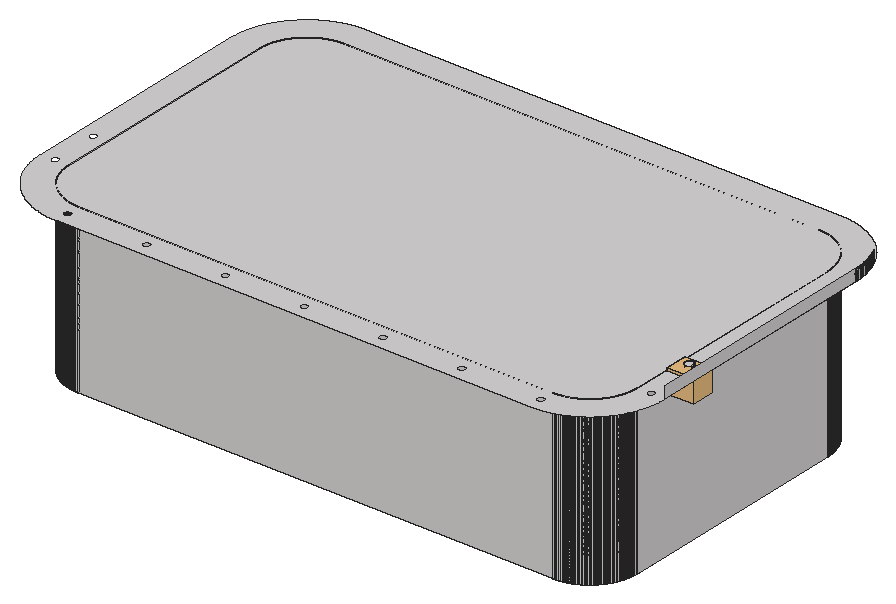
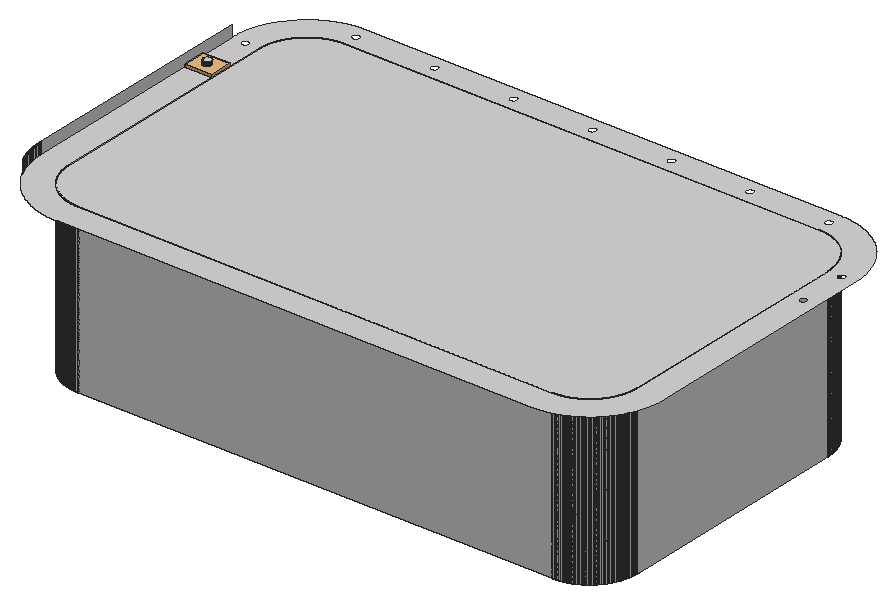
# SketchUp Ruby script. Lengths in inches.
U = 1.inch
M = Sketchup.active_model
def pt(a) = Geom::Point3d.new(a.map { |v| v * U })
def face(e, loops, mat)
  f = e.add_face(loops[0].map { |a| pt(a) })
  loops[1..].each { |l| e.add_face(l.map { |a| pt(a) }).erase! }
  f.material = f.back_material = mat if mat
  f
end
# faces: each face lists its corners as indices into pts; further lists are holes
def faces(e, pts, list, mat = nil) = list.each { |f| face(e, (f[0].is_a?(Array) ? f : [f]).map { |l| l.map { |i| pts[i] } }, mat) }
# xy, xz, yz: faces in a plane at the given z, y or x. An outline is a flat list of corners, or four numbers for a rectangle; further outlines are holes
def ring(l) = l.size == 4 ? [[l[0], l[1]], [l[2], l[1]], [l[2], l[3]], [l[0], l[3]]] : l.each_slice(2).to_a
def flat(e, list, mat, &to3) = list.each { |f| face(e, (f[0].is_a?(Array) ? f : [f]).map { |l| ring(l).map { |u, v| to3.(u, v) } }, mat) }
def xy(e, z, list, mat = nil) = flat(e, list, mat) { |x, y| [x, y, z] }
def xz(e, y, list, mat = nil) = flat(e, list, mat) { |x, z| [x, y, z] }
def yz(e, x, list, mat = nil) = flat(e, list, mat) { |y, z| [x, y, z] }
def lines(e, pts, list) = list.each { |a, b| e.add_line(pt(pts[a]), pt(pts[b])) }
# prism: a flat outline (further loops are holes) pulled along v
def prism(e, loops, v, mat = nil)
  f = face(e, loops, mat); d = Geom::Vector3d.new(v.map { |x| x * U })
  f.pushpull(f.normal.samedirection?(d) ? d.length : -d.length)
end
def box(e, o, s, mat = nil) = prism(e, [[o, [o[0] + s[0], o[1], o[2]], [o[0] + s[0], o[1] + s[1], o[2]], [o[0], o[1] + s[1], o[2]]]], [0, 0, s[2]], mat)
def at(x, y, z, deg = 0) = Geom::Transformation.translation(pt([x, y, z])) * Geom::Transformation.rotation(ORIGIN, Z_AXIS, deg.degrees)
def axes(o, x, y, z) = Geom::Transformation.new([*x, 0, *y, 0, *z, 0, *pt(o).to_a, 1])
def part(name) = M.definitions.add(name)
# library, detail: a bought-in or finely detailed component or shape, given as its bounding box
def library(name, o, s) = part(name).tap { |d| box(d.entities, o, s) }
def detail(e, o, s) = box(e.add_group.entities, o, s)
def put(e, d, t, mat = nil) = e.add_instance(d, t).tap { |i| i.material = mat if mat }
def group(e, t, mat = nil) = e.add_group.tap { |g| g.transformation = t; g.material = mat if mat }.entities
root = M.entities
M.materials.add("[Quartz Light Brown]").color = [215, 212, 212]
c1 = library("3",[-5.26,-4.28,-11.86],[13.52,11.56,11.86])
xy(root,480,[[[224.5,282.7,224.01,282.71,223.01,282.75,222.51,282.78,222.02,282.82,221.52,282.86,221.03,282.91,220.53,282.96,220.04,283.03,219.55,283.09,219.06,283.17,218.56,283.25,218.08,283.34,217.59,283.43,217.1,283.53,216.61,283.64,216.13,283.75,215.65,283.87,215.16,284,214.69,284.13,213.73,284.41,213.26,284.5625,212.79,284.72,212.32,284.88,211.38,285.22,210.92,285.41,210.46,285.59,209.54,285.99,209.09,286.19,208.64,286.4,208.19,286.62,207.75,286.84,207.31,287.07,206.43,287.55,206,287.79,205.57,288.04,205.15,288.3,204.72,288.5625,204.3,288.83,203.89,289.11,203.48,289.38,202.66,289.96,202.26,290.25,201.87,290.55,201.47,290.86,201.09,291.17,200.7,291.49,199.94,292.13,199.57,292.46,199.21,292.8,198.84,293.14,198.48,293.48,197.78,294.18,197.4375,294.54,197.1,294.91,196.76,295.27,196.43,295.65,196.1,296.02,195.78,296.4,194.85,297.57,194.55,297.96,194.26,298.37,193.97,298.77,193.68,299.18,193.4,299.59,193.13,300,192.86,300.42,192.6,300.85,192.34,301.27,192.09,301.7,191.85,302.13,191.6,302.57,191.14,303.45,190.92,303.89,190.7,304.34,190.49,304.79,190.29,305.25,190.09,305.7,189.89,306.16,189.71,306.62,189.52,307.08,189.18,308.02,188.86,308.96,188.71,309.43,188.56,309.91,188.43,310.39,188.29,310.87,188.05,311.83,187.9375,312.31,187.83,312.8,187.73,313.29,187.55,314.27,187.39,315.25,187.33,315.74,187.26,316.23,187.21,316.73,187.16,317.22,187.08,318.22,187.05,318.71,187.01,319.71,187,320.2,187,441.2,187.01,441.7,187.03,442.19,187.05,442.69,187.08,443.1875,187.12,443.68,187.16,444.18,187.21,444.67,187.26,445.17,187.33,445.66,187.39,446.15,187.47,446.65,187.55,447.14,187.73,448.11,187.83,448.6,187.9375,449.09,188.05,449.57,188.17,450.05,188.29,450.54,188.43,451.02,188.56,451.49,188.71,451.97,188.86,452.44,189.02,452.92,189.18,453.39,189.35,453.85,189.52,454.32,189.71,454.78,189.89,455.24,190.29,456.16,190.49,456.61,190.7,457.06,190.92,457.51,191.14,457.95,191.6,458.83,191.85,459.27,192.09,459.7,192.34,460.13,192.6,460.56,192.86,460.98,193.13,461.4,193.4,461.8125,193.68,462.22,194.26,463.04,194.55,463.4375,194.85,463.83,195.16,464.23,195.47,464.62,195.78,465,196.1,465.38,196.43,465.76,196.76,466.13,197.1,466.5,197.4375,466.86,197.78,467.22,198.48,467.92,198.84,468.27,199.21,468.61,199.57,468.94,199.94,469.27,200.32,469.6,200.7,469.92,201.09,470.23,201.47,470.54,201.87,470.85,202.26,471.15,202.66,471.44,203.48,472.02,203.89,472.3,204.3,472.57,204.72,472.84,205.15,473.1,205.57,473.36,206.43,473.86,206.87,474.1,207.75,474.56,208.19,474.78,208.64,475,209.54,475.42,210,475.62,210.92,476,211.38,476.18,212.32,476.52,213.26,476.84,213.73,476.99,214.21,477.14,214.69,477.27,215.16,477.41,215.65,477.53,216.13,477.65,216.61,477.76,217.1,477.87,217.59,477.97,218.08,478.06,218.56,478.15,219.06,478.23,219.55,478.31,220.04,478.375,220.53,478.4375,221.03,478.49,221.52,478.54,222.02,478.58,222.51,478.62,223.01,478.65,223.51,478.67,224.01,478.6875,224.5,478.7,464.5,478.7,464.99,478.6875,465.49,478.67,465.99,478.65,466.49,478.62,466.98,478.58,467.48,478.54,467.97,478.49,468.47,478.4375,468.96,478.375,469.45,478.31,469.94,478.23,470.44,478.15,470.92,478.06,471.41,477.97,471.9,477.87,472.39,477.76,472.87,477.65,473.35,477.53,473.84,477.41,474.31,477.27,474.79,477.14,475.27,476.99,475.74,476.84,476.68,476.52,477.62,476.18,478.08,476,479,475.62,479.46,475.42,480.36,475,480.81,474.78,481.25,474.56,482.13,474.1,482.57,473.86,483.43,473.36,483.85,473.1,484.28,472.84,484.7,472.57,485.11,472.3,485.52,472.02,486.34,471.44,486.74,471.15,487.13,470.85,487.53,470.54,487.91,470.23,488.3,469.92,488.68,469.6,489.06,469.27,489.43,468.94,489.79,468.61,490.16,468.27,490.52,467.92,491.22,467.22,491.5625,466.86,491.9,466.5,492.24,466.13,492.57,465.76,492.9,465.38,493.22,465,493.53,464.62,493.84,464.23,494.15,463.83,494.45,463.4375,494.74,463.04,495.32,462.22,495.6,461.8125,495.87,461.4,496.14,460.98,496.4,460.56,496.66,460.13,496.91,459.7,497.15,459.27,497.4,458.83,497.86,457.95,498.08,457.51,498.3,457.06,498.51,456.61,498.71,456.16,499.11,455.24,499.29,454.78,499.48,454.32,499.65,453.85,499.82,453.39,499.98,452.92,500.14,452.44,500.29,451.97,500.44,451.49,500.57,451.02,500.71,450.54,500.83,450.05,500.95,449.57,501.0625,449.09,501.17,448.6,501.27,448.11,501.45,447.14,501.53,446.65,501.61,446.15,501.67,445.66,501.74,445.17,501.79,444.67,501.84,444.18,501.88,443.68,501.92,443.1875,501.95,442.69,501.97,442.19,501.99,441.7,502,441.2,502,320.2,501.99,319.71,501.95,318.71,501.92,318.22,501.84,317.22,501.79,316.73,501.74,316.23,501.67,315.74,501.61,315.25,501.45,314.27,501.27,313.29,501.17,312.8,501.0625,312.31,500.95,311.83,500.71,310.87,500.57,310.39,500.44,309.91,500.29,309.43,500.14,308.96,499.82,308.02,499.48,307.08,499.29,306.62,499.11,306.16,498.91,305.7,498.71,305.25,498.51,304.79,498.3,304.34,498.08,303.89,497.86,303.45,497.4,302.57,497.15,302.13,496.91,301.7,496.66,301.27,496.4,300.85,496.14,300.42,495.87,300,495.6,299.59,495.32,299.18,495.03,298.77,494.74,298.37,494.45,297.96,494.15,297.57,493.22,296.4,492.9,296.02,492.57,295.65,492.24,295.27,491.9,294.91,491.5625,294.54,491.22,294.18,490.52,293.48,490.16,293.14,489.79,292.8,489.43,292.46,489.06,292.13,488.3,291.49,487.91,291.17,487.53,290.86,487.13,290.55,486.74,290.25,486.34,289.96,485.52,289.38,485.11,289.11,484.7,288.83,484.28,288.5625,483.85,288.3,483.43,288.04,483,287.79,482.57,287.55,481.69,287.07,481.25,286.84,480.81,286.62,480.36,286.4,479.91,286.19,479.46,285.99,478.54,285.59,478.08,285.41,477.62,285.22,476.68,284.88,476.21,284.72,475.74,284.5625,475.27,284.41,474.31,284.13,473.84,284,473.35,283.87,472.87,283.75,472.39,283.64,471.9,283.53,471.41,283.43,470.92,283.34,470.44,283.25,469.94,283.17,469.45,283.09,468.96,283.03,468.47,282.96,467.97,282.91,467.48,282.86,466.98,282.82,466.49,282.78,465.99,282.75,464.99,282.71,464.5,282.7],[494.91,342.7,495.0625,342.7,495.22,342.71,495.53,342.77,495.68,342.82,495.82,342.88,495.96,342.95,496.1,343.03,496.23,343.12,496.35,343.22,496.46,343.33,496.56,343.45,496.74,343.71,496.81,343.85,496.87,343.99,496.92,344.14,496.96,344.29,497,344.61,497,344.76,496.99,344.92,496.96,345.08,496.93,345.23,496.88,345.38,496.82,345.52,496.75,345.66,496.67,345.8,496.58,345.93,496.48,346.05,496.37,346.16,496.25,346.26,496.125,346.35,495.99,346.4375,495.85,346.51,495.71,346.57,495.56,346.62,495.41,346.66,495.25,346.69,495.09,346.7,494.9375,346.7,494.78,346.6875,494.625,346.67,494.47,346.63,494.32,346.58,494.18,346.52,494.04,346.45,493.9,346.37,493.77,346.28,493.65,346.18,493.54,346.07,493.44,345.95,493.35,345.83,493.26,345.69,493.19,345.55,493.13,345.41,493.08,345.26,493.04,345.11,493.02,344.95,493,344.8,493,344.64,493.01,344.48,493.04,344.33,493.07,344.17,493.12,344.02,493.18,343.88,493.25,343.74,493.33,343.6,493.42,343.48,493.52,343.36,493.63,343.24,493.75,343.14,493.875,343.05,494.01,342.96,494.15,342.89,494.29,342.83,494.44,342.78,494.59,342.74],[494.91,318.7,495.0625,318.7,495.22,318.71,495.53,318.77,495.68,318.82,495.82,318.88,495.96,318.95,496.1,319.03,496.23,319.12,496.35,319.22,496.46,319.33,496.56,319.45,496.74,319.71,496.81,319.85,496.87,319.99,496.92,320.14,496.96,320.29,497,320.61,497,320.76,496.99,320.92,496.96,321.08,496.93,321.23,496.88,321.38,496.82,321.52,496.75,321.66,496.67,321.8,496.58,321.93,496.48,322.05,496.37,322.16,496.25,322.26,496.125,322.35,495.99,322.4375,495.85,322.51,495.71,322.57,495.56,322.62,495.41,322.66,495.25,322.69,495.09,322.7,494.9375,322.7,494.78,322.6875,494.625,322.67,494.47,322.63,494.32,322.58,494.18,322.52,494.04,322.45,493.9,322.37,493.77,322.28,493.65,322.18,493.54,322.07,493.44,321.95,493.35,321.83,493.26,321.69,493.19,321.55,493.13,321.41,493.08,321.26,493.04,321.11,493.02,320.95,493,320.8,493,320.64,493.01,320.48,493.04,320.33,493.07,320.17,493.12,320.02,493.18,319.88,493.25,319.74,493.33,319.6,493.42,319.48,493.52,319.36,493.63,319.24,493.75,319.14,493.875,319.05,494.01,318.96,494.15,318.89,494.29,318.83,494.44,318.78,494.59,318.74],[224.9375,287.7,225.09,287.7,225.41,287.74,225.56,287.78,225.71,287.83,225.85,287.89,225.99,287.96,226.125,288.05,226.25,288.14,226.37,288.24,226.48,288.36,226.58,288.48,226.67,288.6,226.75,288.74,226.82,288.88,226.88,289.02,226.93,289.17,226.96,289.33,226.99,289.48,227,289.64,227,289.8,226.98,289.95,226.96,290.11,226.92,290.26,226.87,290.41,226.81,290.55,226.74,290.69,226.65,290.83,226.56,290.95,226.46,291.07,226.35,291.18,226.23,291.28,226.1,291.37,225.96,291.45,225.82,291.52,225.68,291.58,225.53,291.63,225.375,291.67,225.22,291.6875,225.0625,291.7,224.91,291.7,224.75,291.69,224.59,291.66,224.44,291.62,224.29,291.57,224.15,291.51,224.01,291.4375,223.875,291.35,223.75,291.26,223.63,291.16,223.52,291.05,223.42,290.93,223.33,290.8,223.25,290.66,223.18,290.52,223.12,290.38,223.07,290.23,223.04,290.08,223.01,289.92,223,289.76,223,289.61,223.04,289.29,223.08,289.14,223.13,288.99,223.19,288.85,223.26,288.71,223.44,288.45,223.54,288.33,223.65,288.22,223.77,288.12,223.9,288.03,224.04,287.95,224.18,287.88,224.32,287.82,224.47,287.77,224.78,287.71],[264.77,287.7,264.93,287.7,265.08,287.72,265.24,287.74,265.39,287.78,265.54,287.83,265.69,287.89,265.82,287.96,265.96,288.05,266.08,288.14,266.2,288.24,266.3125,288.36,266.41,288.48,266.51,288.6,266.59,288.74,266.66,288.88,266.72,289.02,266.76,289.17,266.8,289.33,266.82,289.48,266.83,289.64,266.83,289.8,266.82,289.95,266.79,290.11,266.75,290.26,266.7,290.41,266.64,290.55,266.57,290.69,266.49,290.83,266.29,291.07,266.18,291.18,266.06,291.28,265.93,291.37,265.8,291.45,265.66,291.52,265.51,291.58,265.36,291.63,265.21,291.67,265.05,291.6875,264.9,291.7,264.74,291.7,264.58,291.69,264.43,291.66,264.27,291.62,264.125,291.57,263.98,291.51,263.84,291.4375,263.71,291.35,263.58,291.26,263.46,291.16,263.35,291.05,263.25,290.93,263.16,290.8,263.08,290.66,263.01,290.52,262.95,290.38,262.9,290.23,262.87,290.08,262.83,289.76,262.84,289.61,262.85,289.45,262.875,289.29,262.91,289.14,262.96,288.99,263.02,288.85,263.1,288.71,263.18,288.58,263.27,288.45,263.375,288.33,263.49,288.22,263.61,288.12,263.74,288.03,263.87,287.95,264.01,287.88,264.16,287.82,264.31,287.77,264.61,287.71],[304.6,287.7,304.76,287.7,304.92,287.72,305.07,287.74,305.23,287.78,305.375,287.83,305.52,287.89,305.66,287.96,305.92,288.14,306.04,288.24,306.15,288.36,306.25,288.48,306.34,288.6,306.42,288.74,306.49,288.88,306.55,289.02,306.6,289.17,306.63,289.33,306.65,289.48,306.67,289.64,306.66,289.8,306.65,289.95,306.625,290.11,306.59,290.26,306.54,290.41,306.48,290.55,306.32,290.83,306.23,290.95,306.125,291.07,306.01,291.18,305.89,291.28,305.76,291.37,305.63,291.45,305.49,291.52,305.34,291.58,305.19,291.63,305.04,291.67,304.89,291.6875,304.73,291.7,304.57,291.7,304.42,291.69,304.26,291.66,304.11,291.62,303.96,291.57,303.81,291.51,303.68,291.4375,303.54,291.35,303.42,291.26,303.3,291.16,303.1875,291.05,303.09,290.93,302.99,290.8,302.91,290.66,302.84,290.52,302.78,290.38,302.7,290.08,302.68,289.92,302.67,289.76,302.67,289.61,302.68,289.45,302.71,289.29,302.75,289.14,302.8,288.99,302.86,288.85,302.93,288.71,303.01,288.58,303.11,288.45,303.21,288.33,303.32,288.22,303.44,288.12,303.57,288.03,303.7,287.95,303.84,287.88,303.99,287.82,304.14,287.77,304.29,287.74,304.45,287.71],[344.4375,287.7,344.59,287.7,344.91,287.74,345.06,287.78,345.21,287.83,345.35,287.89,345.49,287.96,345.625,288.05,345.75,288.14,345.87,288.24,345.98,288.36,346.08,288.48,346.17,288.6,346.25,288.74,346.32,288.88,346.38,289.02,346.43,289.17,346.46,289.33,346.49,289.48,346.5,289.64,346.5,289.8,346.48,289.95,346.46,290.11,346.42,290.26,346.37,290.41,346.31,290.55,346.24,290.69,346.15,290.83,346.06,290.95,345.96,291.07,345.85,291.18,345.73,291.28,345.6,291.37,345.46,291.45,345.32,291.52,345.18,291.58,345.03,291.63,344.875,291.67,344.72,291.6875,344.5625,291.7,344.41,291.7,344.25,291.69,344.09,291.66,343.94,291.62,343.79,291.57,343.65,291.51,343.51,291.4375,343.375,291.35,343.25,291.26,343.13,291.16,343.02,291.05,342.92,290.93,342.83,290.8,342.75,290.66,342.68,290.52,342.62,290.38,342.57,290.23,342.54,290.08,342.51,289.92,342.5,289.76,342.5,289.61,342.54,289.29,342.58,289.14,342.63,288.99,342.69,288.85,342.76,288.71,342.94,288.45,343.04,288.33,343.15,288.22,343.27,288.12,343.4,288.03,343.54,287.95,343.68,287.88,343.82,287.82,343.97,287.77,344.28,287.71],[384.27,287.7,384.43,287.7,384.58,287.72,384.74,287.74,384.89,287.78,385.04,287.83,385.19,287.89,385.32,287.96,385.46,288.05,385.58,288.14,385.7,288.24,385.8125,288.36,385.91,288.48,386.01,288.6,386.09,288.74,386.16,288.88,386.22,289.02,386.26,289.17,386.3,289.33,386.32,289.48,386.33,289.64,386.33,289.8,386.32,289.95,386.29,290.11,386.25,290.26,386.2,290.41,386.14,290.55,386.07,290.69,385.99,290.83,385.79,291.07,385.68,291.18,385.56,291.28,385.43,291.37,385.3,291.45,385.16,291.52,385.01,291.58,384.86,291.63,384.71,291.67,384.55,291.6875,384.4,291.7,384.24,291.7,384.08,291.69,383.93,291.66,383.77,291.62,383.625,291.57,383.48,291.51,383.34,291.4375,383.21,291.35,383.08,291.26,382.96,291.16,382.85,291.05,382.75,290.93,382.66,290.8,382.58,290.66,382.51,290.52,382.45,290.38,382.4,290.23,382.37,290.08,382.33,289.76,382.34,289.61,382.35,289.45,382.375,289.29,382.41,289.14,382.46,288.99,382.52,288.85,382.6,288.71,382.68,288.58,382.77,288.45,382.875,288.33,382.99,288.22,383.11,288.12,383.24,288.03,383.37,287.95,383.51,287.88,383.66,287.82,383.81,287.77,384.11,287.71],[424.1,287.7,424.26,287.7,424.42,287.72,424.57,287.74,424.73,287.78,424.875,287.83,425.02,287.89,425.16,287.96,425.42,288.14,425.54,288.24,425.65,288.36,425.75,288.48,425.84,288.6,425.92,288.74,425.99,288.88,426.05,289.02,426.1,289.17,426.13,289.33,426.15,289.48,426.17,289.64,426.16,289.8,426.15,289.95,426.125,290.11,426.09,290.26,426.04,290.41,425.98,290.55,425.82,290.83,425.73,290.95,425.625,291.07,425.51,291.18,425.39,291.28,425.26,291.37,425.13,291.45,424.99,291.52,424.84,291.58,424.69,291.63,424.54,291.67,424.39,291.6875,424.23,291.7,424.07,291.7,423.92,291.69,423.76,291.66,423.61,291.62,423.46,291.57,423.31,291.51,423.18,291.4375,423.04,291.35,422.92,291.26,422.8,291.16,422.6875,291.05,422.59,290.93,422.49,290.8,422.41,290.66,422.34,290.52,422.28,290.38,422.2,290.08,422.18,289.92,422.17,289.76,422.17,289.61,422.18,289.45,422.21,289.29,422.25,289.14,422.3,288.99,422.36,288.85,422.43,288.71,422.51,288.58,422.61,288.45,422.71,288.33,422.82,288.22,422.94,288.12,423.07,288.03,423.2,287.95,423.34,287.88,423.49,287.82,423.64,287.77,423.79,287.74,423.95,287.71],[463.9375,287.7,464.09,287.7,464.41,287.74,464.56,287.78,464.71,287.83,464.85,287.89,464.99,287.96,465.125,288.05,465.25,288.14,465.37,288.24,465.48,288.36,465.58,288.48,465.67,288.6,465.75,288.74,465.82,288.88,465.88,289.02,465.93,289.17,465.96,289.33,465.99,289.48,466,289.64,466,289.8,465.98,289.95,465.96,290.11,465.92,290.26,465.87,290.41,465.81,290.55,465.74,290.69,465.65,290.83,465.56,290.95,465.46,291.07,465.35,291.18,465.23,291.28,465.1,291.37,464.96,291.45,464.82,291.52,464.68,291.58,464.53,291.63,464.375,291.67,464.22,291.6875,464.0625,291.7,463.91,291.7,463.75,291.69,463.59,291.66,463.44,291.62,463.29,291.57,463.15,291.51,463.01,291.4375,462.875,291.35,462.75,291.26,462.63,291.16,462.52,291.05,462.42,290.93,462.33,290.8,462.25,290.66,462.18,290.52,462.12,290.38,462.07,290.23,462.04,290.08,462.01,289.92,462,289.76,462,289.61,462.04,289.29,462.08,289.14,462.13,288.99,462.19,288.85,462.26,288.71,462.44,288.45,462.54,288.33,462.65,288.22,462.77,288.12,462.9,288.03,463.04,287.95,463.18,287.88,463.32,287.82,463.47,287.77,463.78,287.71],[193.9375,318.7,194.09,318.7,194.41,318.74,194.56,318.78,194.71,318.83,194.85,318.89,194.99,318.96,195.125,319.05,195.25,319.14,195.37,319.24,195.48,319.36,195.58,319.48,195.67,319.6,195.75,319.74,195.82,319.88,195.88,320.02,195.93,320.17,195.96,320.33,195.99,320.48,196,320.64,196,320.8,195.98,320.95,195.96,321.11,195.92,321.26,195.87,321.41,195.81,321.55,195.74,321.69,195.65,321.83,195.56,321.95,195.46,322.07,195.35,322.18,195.23,322.28,195.1,322.37,194.96,322.45,194.82,322.52,194.68,322.58,194.53,322.63,194.375,322.67,194.22,322.6875,194.0625,322.7,193.91,322.7,193.75,322.69,193.59,322.66,193.44,322.62,193.29,322.57,193.15,322.51,193.01,322.4375,192.875,322.35,192.75,322.26,192.63,322.16,192.52,322.05,192.42,321.93,192.33,321.8,192.25,321.66,192.18,321.52,192.12,321.38,192.07,321.23,192.04,321.08,192.01,320.92,192,320.76,192,320.61,192.04,320.29,192.08,320.14,192.13,319.99,192.19,319.85,192.26,319.71,192.44,319.45,192.54,319.33,192.65,319.22,192.77,319.12,192.9,319.03,193.04,318.95,193.18,318.88,193.32,318.82,193.47,318.77,193.78,318.71],[193.9375,342.7,194.09,342.7,194.41,342.74,194.56,342.78,194.71,342.83,194.85,342.89,194.99,342.96,195.125,343.05,195.25,343.14,195.37,343.24,195.48,343.36,195.58,343.48,195.67,343.6,195.75,343.74,195.82,343.88,195.88,344.02,195.93,344.17,195.96,344.33,195.99,344.48,196,344.64,196,344.8,195.98,344.95,195.96,345.11,195.92,345.26,195.87,345.41,195.81,345.55,195.74,345.69,195.65,345.83,195.56,345.95,195.46,346.07,195.35,346.18,195.23,346.28,195.1,346.37,194.96,346.45,194.82,346.52,194.68,346.58,194.53,346.63,194.375,346.67,194.22,346.6875,194.0625,346.7,193.91,346.7,193.75,346.69,193.59,346.66,193.44,346.62,193.29,346.57,193.15,346.51,193.01,346.4375,192.875,346.35,192.75,346.26,192.63,346.16,192.52,346.05,192.42,345.93,192.33,345.8,192.25,345.66,192.18,345.52,192.12,345.38,192.07,345.23,192.04,345.08,192.01,344.92,192,344.76,192,344.61,192.04,344.29,192.08,344.14,192.13,343.99,192.19,343.85,192.26,343.71,192.44,343.45,192.54,343.33,192.65,343.22,192.77,343.12,192.9,343.03,193.04,342.95,193.18,342.88,193.32,342.82,193.47,342.77,193.78,342.71]]],"[Quartz Light Brown]")
xy(root,483,[[494.91,342.7,494.59,342.74,494.44,342.78,494.29,342.83,494.15,342.89,494.01,342.96,493.875,343.05,493.75,343.14,493.63,343.24,493.52,343.36,493.42,343.48,493.33,343.6,493.25,343.74,493.18,343.88,493.12,344.02,493.07,344.17,493.04,344.33,493.01,344.48,493,344.64,493,344.8,493.02,344.95,493.04,345.11,493.08,345.26,493.13,345.41,493.19,345.55,493.26,345.69,493.35,345.83,493.44,345.95,493.54,346.07,493.65,346.18,493.77,346.28,493.9,346.37,494.04,346.45,494.18,346.52,494.32,346.58,494.47,346.63,494.625,346.67,494.78,346.6875,494.9375,346.7,495.09,346.7,495.25,346.69,495.41,346.66,495.56,346.62,495.71,346.57,495.85,346.51,495.99,346.4375,496.125,346.35,496.25,346.26,496.37,346.16,496.48,346.05,496.58,345.93,496.67,345.8,496.75,345.66,496.82,345.52,496.88,345.38,496.93,345.23,496.96,345.08,496.99,344.92,497,344.76,497,344.61,496.96,344.29,496.92,344.14,496.87,343.99,496.81,343.85,496.74,343.71,496.56,343.45,496.46,343.33,496.35,343.22,496.23,343.12,496.1,343.03,495.96,342.95,495.82,342.88,495.68,342.82,495.53,342.77,495.22,342.71,495.0625,342.7]],"[Quartz Light Brown]")
xz(root,346.7,[[494.9375,480,495.09,483]],"[Quartz Light Brown]")
yz(root,493,[[344.64,480,344.8,483]],"[Quartz Light Brown]")
yz(root,497,[[344.61,480,344.76,483]],"[Quartz Light Brown]")
yz(root,502,[[320.7,480,440.7,486],[440.7,480,441.2,486]],"[Quartz Light Brown]")
p = [[496.96,344.29,480],[496.92,344.14,480],[496.92,344.14,483],[496.96,344.29,483],[493.07,344.17,480],[493.04,344.33,480],
  [493.04,344.33,483],[493.07,344.17,483],[493.01,344.48,480],[493.01,344.48,483],[496.98,344.45,480],[496.98,344.45,483],
  [497,344.61,480],[497,344.61,483],[493,344.64,480],[493,344.64,483],[493,344.8,480],[493.02,344.95,480],
  [493.02,344.95,483],[493,344.8,483],[496.99,344.92,480],[497,344.76,480],[497,344.76,483],[496.99,344.92,483],
  [496.96,345.08,480],[496.96,345.08,483],[493.04,345.11,480],[493.04,345.11,483],[493.08,345.26,480],[493.08,345.26,483],
  [496.93,345.23,480],[496.93,345.23,483],[496.88,345.38,480],[496.88,345.38,483],[493.13,345.41,480],[493.13,345.41,483],
  [493.19,345.55,480],[493.19,345.55,483],[496.82,345.52,480],[496.82,345.52,483],[496.75,345.66,480],[496.75,345.66,483],
  [493.26,345.69,480],[493.26,345.69,483],[493.35,345.83,480],[493.35,345.83,483],[496.67,345.8,480],[496.67,345.8,483],
  [493.44,345.95,480],[493.44,345.95,483],[496.58,345.93,480],[496.58,345.93,483],[496.48,346.05,480],[496.48,346.05,483],
  [493.54,346.07,480],[493.54,346.07,483],[496.37,346.16,480],[496.37,346.16,483],[493.65,346.18,480],[493.65,346.18,483],
  [493.77,346.28,480],[493.77,346.28,483],[496.25,346.26,480],[496.25,346.26,483],[493.9,346.37,480],[493.9,346.37,483],
  [496.125,346.35,480],[496.125,346.35,483],[494.04,346.45,480],[494.04,346.45,483],[495.85,346.51,480],[495.99,346.4375,480],
  [495.99,346.4375,483],[495.85,346.51,483],[494.18,346.52,480],[494.18,346.52,483],[494.32,346.58,480],[494.32,346.58,483],
  [495.71,346.57,480],[495.71,346.57,483],[494.47,346.63,480],[494.47,346.63,483],[494.625,346.67,480],[494.625,346.67,483],
  [495.41,346.66,480],[495.56,346.62,480],[495.56,346.62,483],[495.41,346.66,483],[494.78,346.6875,480],[494.78,346.6875,483],
  [494.9375,346.7,480],[494.9375,346.7,483],[495.09,346.7,480],[495.25,346.69,480],[495.25,346.69,483],[495.09,346.7,483],
  [502,441.2,480],[501.99,441.7,480],[501.99,441.7,486],[502,441.2,486],[501.97,442.19,480],[501.97,442.19,486],
  [501.95,442.69,480],[501.95,442.69,486],[501.92,443.1875,480],[501.92,443.1875,486],[501.88,443.68,480],[501.88,443.68,486],
  [501.84,444.18,480],[501.84,444.18,486],[501.79,444.67,480],[501.79,444.67,486],[501.74,445.17,480],[501.74,445.17,486],
  [501.67,445.66,480],[501.67,445.66,486],[501.61,446.15,480],[501.61,446.15,486],[501.53,446.65,480],[501.53,446.65,486],
  [501.45,447.14,480],[501.45,447.14,486],[501.36,447.625,480],[501.36,447.625,486],[501.27,448.11,480],[501.27,448.11,486],
  [501.17,448.6,480],[501.17,448.6,486],[501.0625,449.09,480],[501.0625,449.09,486],[500.95,449.57,480],[500.95,449.57,486],
  [500.83,450.05,480],[500.83,450.05,486],[500.71,450.54,480],[500.71,450.54,486],[500.57,451.02,480],[500.57,451.02,486],
  [500.44,451.49,480],[500.44,451.49,486],[500.29,451.97,480],[500.29,451.97,486],[500.14,452.44,480],[500.14,452.44,486],
  [499.98,452.92,480],[499.98,452.92,486],[499.82,453.39,480],[499.82,453.39,486],[499.65,453.85,480],[499.65,453.85,486],
  [499.48,454.32,480],[499.48,454.32,486],[499.29,454.78,480],[499.29,454.78,486],[499.11,455.24,480],[499.11,455.24,486],
  [498.91,455.7,480],[498.91,455.7,486],[498.71,456.16,480],[498.71,456.16,486],[498.51,456.61,480],[498.51,456.61,486],
  [498.3,457.06,480],[498.3,457.06,486],[498.08,457.51,480],[498.08,457.51,486]]
faces(root,p,[[0,1,2,3],[4,5,6,7],[5,8,9,6],[10,0,3,11],[12,10,11,13],[8,14,15,9],[16,17,18,19],[20,21,22,23],
  [24,20,23,25],[17,26,27,18],[26,28,29,27],[30,24,25,31],[32,30,31,33],[28,34,35,29],[34,36,37,35],[38,32,33,39],
  [40,38,39,41],[36,42,43,37],[42,44,45,43],[46,40,41,47],[44,48,49,45],[50,46,47,51],[52,50,51,53],[48,54,55,49],
  [56,52,53,57],[54,58,59,55],[58,60,61,59],[62,56,57,63],[60,64,65,61],[66,62,63,67],[64,68,69,65],[70,71,72,73],
  [71,66,67,72],[68,74,75,69],[74,76,77,75],[78,70,73,79],[76,80,81,77],[80,82,83,81],[84,85,86,87],[85,78,79,86],
  [82,88,89,83],[88,90,91,89],[92,93,94,95],[93,84,87,94],[96,97,98,99],[97,100,101,98],[100,102,103,101],[102,104,105,103],
  [104,106,107,105],[106,108,109,107],[108,110,111,109],[110,112,113,111],[112,114,115,113],[114,116,117,115],[116,118,119,117],[118,120,121,119],
  [120,122,123,121],[122,124,125,123],[124,126,127,125],[126,128,129,127],[128,130,131,129],[130,132,133,131],[132,134,135,133],[134,136,137,135],
  [136,138,139,137],[138,140,141,139],[140,142,143,141],[142,144,145,143],[144,146,147,145],[146,148,149,147],[148,150,151,149],[150,152,153,151],
  [152,154,155,153],[154,156,157,155],[156,158,159,157],[158,160,161,159],[160,162,163,161],[162,164,165,163]],"[Quartz Light Brown]")
put(root,c1,axes([496.5,343.2,481.25],[-1,0,0],[0,1,0],[0,0,1]),"[Quartz Light Brown]")
g1 = group(root,at(201,296.68,396),"[Quartz Light Brown]")
prism(g1,[[[263,0,0],[24,0,0],[23.6875,0,0],[23.37,0.01,0],[23.06,0.02,0],[22.74,0.03,0],[22.43,0.05,0],[22.12,0.07,0],[21.8,0.1,0],[21.49,0.13,0],[21.18,0.17,0],[20.87,0.21,0],[20.56,0.25,0],[20.25,0.3,0],[19.9375,0.35,0],[19.625,0.4,0],[19.32,0.46,0],[19.01,0.52,0],[18.7,0.59,0],[18.4,0.66,0],[18.09,0.74,0],[17.79,0.82,0],[17.49,0.9,0],[17.18,0.99,0],[16.88,1.08,0],[16.58,1.17,0],[16.29,1.27,0],[15.99,1.375,0],[15.69,1.48,0],[15.4,1.59,0],[15.11,1.71,0],[14.82,1.83,0],[14.53,1.95,0],[14.24,2.07,0],[13.95,2.2,0],[13.67,2.34,0],[13.39,2.48,0],[13.1,2.62,0],[12.83,2.76,0],[12.55,2.91,0],[12.27,3.06,0],[12,3.22,0],[11.73,3.375,0],[11.46,3.54,0],[11.19,3.7,0],[10.93,3.87,0],[10.67,4.04,0],[10.41,4.22,0],[10.15,4.4,0],[9.89,4.58,0],[9.64,4.77,0],[9.39,4.96,0],[9.14,5.15,0],[8.9,5.35,0],[8.65,5.55,0],[8.41,5.75,0],[8.18,5.96,0],[7.94,6.16,0],[7.71,6.375,0],[7.48,6.59,0],[7.25,6.81,0],[7.03,7.03,0],[6.81,7.25,0],[6.59,7.48,0],[6.375,7.71,0],[6.16,7.94,0],[5.96,8.18,0],[5.75,8.41,0],[5.55,8.65,0],[5.35,8.9,0],[5.15,9.14,0],[4.96,9.39,0],[4.77,9.64,0],[4.58,9.89,0],[4.4,10.15,0],[4.22,10.41,0],[4.04,10.67,0],[3.87,10.93,0],[3.7,11.19,0],[3.54,11.46,0],[3.375,11.73,0],[3.22,12,0],[3.06,12.27,0],[2.91,12.55,0],[2.76,12.83,0],[2.62,13.1,0],[2.48,13.39,0],[2.34,13.67,0],[2.2,13.95,0],[2.07,14.24,0],[1.95,14.53,0],[1.83,14.82,0],[1.71,15.11,0],[1.59,15.4,0],[1.48,15.69,0],[1.375,15.99,0],[1.27,16.29,0],[1.17,16.58,0],[1.08,16.88,0],[0.99,17.18,0],[0.9,17.49,0],[0.82,17.79,0],[0.74,18.09,0],[0.66,18.4,0],[0.59,18.7,0],[0.52,19.01,0],[0.46,19.32,0],[0.4,19.625,0],[0.35,19.9375,0],[0.3,20.25,0],[0.25,20.56,0],[0.21,20.87,0],[0.17,21.18,0],[0.13,21.49,0],[0.1,21.8,0],[0.07,22.12,0],[0.05,22.43,0],[0.03,22.74,0],[0.02,23.06,0],[0.01,23.37,0],[0,23.6875,0],[0,24,0],[0,144,0],[0,144.3125,0],[0.01,144.63,0],[0.02,144.94,0],[0.03,145.26,0],[0.05,145.57,0],[0.07,145.88,0],[0.1,146.2,0],[0.13,146.51,0],[0.17,146.82,0],[0.21,147.13,0],[0.25,147.44,0],[0.3,147.75,0],[0.35,148.0625,0],[0.4,148.375,0],[0.46,148.68,0],[0.52,148.99,0],[0.59,149.3,0],[0.66,149.6,0],[0.74,149.91,0],[0.82,150.21,0],[0.9,150.51,0],[0.99,150.82,0],[1.08,151.12,0],[1.17,151.42,0],[1.27,151.71,0],[1.375,152.01,0],[1.48,152.31,0],[1.59,152.6,0],[1.71,152.89,0],[1.83,153.18,0],[1.95,153.47,0],[2.07,153.76,0],[2.2,154.05,0],[2.34,154.33,0],[2.48,154.61,0],[2.62,154.9,0],[2.76,155.17,0],[2.91,155.45,0],[3.06,155.73,0],[3.22,156,0],[3.375,156.27,0],[3.54,156.54,0],[3.7,156.81,0],[3.87,157.07,0],[4.04,157.33,0],[4.22,157.59,0],[4.4,157.85,0],[4.58,158.11,0],[4.77,158.36,0],[4.96,158.61,0],[5.15,158.86,0],[5.35,159.1,0],[5.55,159.35,0],[5.75,159.59,0],[5.96,159.82,0],[6.16,160.06,0],[6.375,160.29,0],[6.59,160.52,0],[6.81,160.75,0],[7.03,160.97,0],[7.25,161.19,0],[7.48,161.41,0],[7.71,161.625,0],[7.94,161.84,0],[8.18,162.04,0],[8.41,162.25,0],[8.65,162.45,0],[8.9,162.65,0],[9.14,162.85,0],[9.39,163.04,0],[9.64,163.23,0],[9.89,163.42,0],[10.15,163.6,0],[10.41,163.78,0],[10.67,163.96,0],[10.93,164.13,0],[11.19,164.3,0],[11.46,164.46,0],[11.73,164.625,0],[12,164.78,0],[12.27,164.94,0],[12.55,165.09,0],[12.83,165.24,0],[13.1,165.38,0],[13.39,165.52,0],[13.67,165.66,0],[13.95,165.8,0],[14.24,165.93,0],[14.53,166.05,0],[14.82,166.17,0],[15.11,166.29,0],[15.4,166.41,0],[15.69,166.52,0],[15.99,166.625,0],[16.29,166.73,0],[16.58,166.83,0],[16.88,166.92,0],[17.18,167.01,0],[17.49,167.1,0],[17.79,167.18,0],[18.09,167.26,0],[18.4,167.34,0],[18.7,167.41,0],[19.01,167.48,0],[19.32,167.54,0],[19.625,167.6,0],[19.9375,167.65,0],[20.25,167.7,0],[20.56,167.75,0],[20.87,167.79,0],[21.18,167.83,0],[21.49,167.87,0],[21.8,167.9,0],[22.12,167.93,0],[22.43,167.95,0],[22.74,167.97,0],[23.06,167.98,0],[23.37,167.99,0],[23.6875,168,0],[24,168,0],[263,168,0],[263.3125,168,0],[263.63,167.99,0],[263.94,167.98,0],[264.26,167.97,0],[264.57,167.95,0],[264.88,167.93,0],[265.2,167.9,0],[265.51,167.87,0],[265.82,167.83,0],[266.13,167.79,0],[266.44,167.75,0],[266.75,167.7,0],[267.0625,167.65,0],[267.375,167.6,0],[267.68,167.54,0],[267.99,167.48,0],[268.3,167.41,0],[268.6,167.34,0],[268.91,167.26,0],[269.21,167.18,0],[269.51,167.1,0],[269.82,167.01,0],[270.12,166.92,0],[270.42,166.83,0],[270.71,166.73,0],[271.01,166.625,0],[271.31,166.52,0],[271.6,166.41,0],[271.89,166.29,0],[272.18,166.17,0],[272.47,166.05,0],[272.76,165.93,0],[273.05,165.8,0],[273.33,165.66,0],[273.61,165.52,0],[273.9,165.38,0],[274.17,165.24,0],[274.45,165.09,0],[274.73,164.94,0],[275,164.78,0],[275.27,164.625,0],[275.54,164.46,0],[275.81,164.3,0],[276.07,164.13,0],[276.33,163.96,0],[276.59,163.78,0],[276.85,163.6,0],[277.11,163.42,0],[277.36,163.23,0],[277.61,163.04,0],[277.86,162.85,0],[278.1,162.65,0],[278.35,162.45,0],[278.59,162.25,0],[278.82,162.04,0],[279.06,161.84,0],[279.29,161.625,0],[279.52,161.41,0],[279.75,161.19,0],[279.97,160.97,0],[280.19,160.75,0],[280.41,160.52,0],[280.625,160.29,0],[280.84,160.06,0],[281.04,159.82,0],[281.25,159.59,0],[281.45,159.35,0],[281.65,159.1,0],[281.85,158.86,0],[282.04,158.61,0],[282.23,158.36,0],[282.42,158.11,0],[282.6,157.85,0],[282.78,157.59,0],[282.96,157.33,0],[283.13,157.07,0],[283.3,156.81,0],[283.46,156.54,0],[283.625,156.27,0],[283.78,156,0],[283.94,155.73,0],[284.09,155.45,0],[284.24,155.17,0],[284.38,154.9,0],[284.52,154.61,0],[284.66,154.33,0],[284.8,154.05,0],[284.93,153.76,0],[285.05,153.47,0],[285.17,153.18,0],[285.29,152.89,0],[285.41,152.6,0],[285.52,152.31,0],[285.625,152.01,0],[285.73,151.71,0],[285.83,151.42,0],[285.92,151.12,0],[286.01,150.82,0],[286.1,150.51,0],[286.18,150.21,0],[286.26,149.91,0],[286.34,149.6,0],[286.41,149.3,0],[286.48,148.99,0],[286.54,148.68,0],[286.6,148.375,0],[286.65,148.0625,0],[286.7,147.75,0],[286.75,147.44,0],[286.79,147.13,0],[286.83,146.82,0],[286.87,146.51,0],[286.9,146.2,0],[286.93,145.88,0],[286.95,145.57,0],[286.97,145.26,0],[286.98,144.94,0],[286.99,144.63,0],[287,144.3125,0],[287,144,0],[287,24,0],[287,23.6875,0],[286.99,23.37,0],[286.98,23.06,0],[286.97,22.74,0],[286.95,22.43,0],[286.93,22.12,0],[286.9,21.8,0],[286.87,21.49,0],[286.83,21.18,0],[286.79,20.87,0],[286.75,20.56,0],[286.7,20.25,0],[286.65,19.9375,0],[286.6,19.625,0],[286.54,19.32,0],[286.48,19.01,0],[286.41,18.7,0],[286.34,18.4,0],[286.26,18.09,0],[286.18,17.79,0],[286.1,17.49,0],[286.01,17.18,0],[285.92,16.88,0],[285.83,16.58,0],[285.73,16.29,0],[285.625,15.99,0],[285.52,15.69,0],[285.41,15.4,0],[285.29,15.11,0],[285.17,14.82,0],[285.05,14.53,0],[284.93,14.24,0],[284.8,13.95,0],[284.66,13.67,0],[284.52,13.39,0],[284.38,13.1,0],[284.24,12.83,0],[284.09,12.55,0],[283.94,12.27,0],[283.78,12,0],[283.625,11.73,0],[283.46,11.46,0],[283.3,11.19,0],[283.13,10.93,0],[282.96,10.67,0],[282.78,10.41,0],[282.6,10.15,0],[282.42,9.89,0],[282.23,9.64,0],[282.04,9.39,0],[281.85,9.14,0],[281.65,8.9,0],[281.45,8.65,0],[281.25,8.41,0],[281.04,8.18,0],[280.84,7.94,0],[280.625,7.71,0],[280.41,7.48,0],[280.19,7.25,0],[279.97,7.03,0],[279.75,6.81,0],[279.52,6.59,0],[279.29,6.375,0],[279.06,6.16,0],[278.82,5.96,0],[278.59,5.75,0],[278.35,5.55,0],[278.1,5.35,0],[277.86,5.15,0],[277.61,4.96,0],[277.36,4.77,0],[277.11,4.58,0],[276.85,4.4,0],[276.59,4.22,0],[276.33,4.04,0],[276.07,3.87,0],[275.81,3.7,0],[275.54,3.54,0],[275.27,3.375,0],[275,3.22,0],[274.73,3.06,0],[274.45,2.91,0],[274.17,2.76,0],[273.9,2.62,0],[273.61,2.48,0],[273.33,2.34,0],[273.05,2.2,0],[272.76,2.07,0],[272.47,1.95,0],[272.18,1.83,0],[271.89,1.71,0],[271.6,1.59,0],[271.31,1.48,0],[271.01,1.375,0],[270.71,1.27,0],[270.42,1.17,0],[270.12,1.08,0],[269.82,0.99,0],[269.51,0.9,0],[269.21,0.82,0],[268.91,0.74,0],[268.6,0.66,0],[268.3,0.59,0],[267.99,0.52,0],[267.68,0.46,0],[267.375,0.4,0],[267.0625,0.35,0],[266.75,0.3,0],[266.44,0.25,0],[266.13,0.21,0],[265.82,0.17,0],[265.51,0.13,0],[265.2,0.1,0],[264.88,0.07,0],[264.57,0.05,0],[264.26,0.03,0],[263.94,0.02,0],[263.63,0.01,0],[263.3125,0,0]]],[0,0,84])
